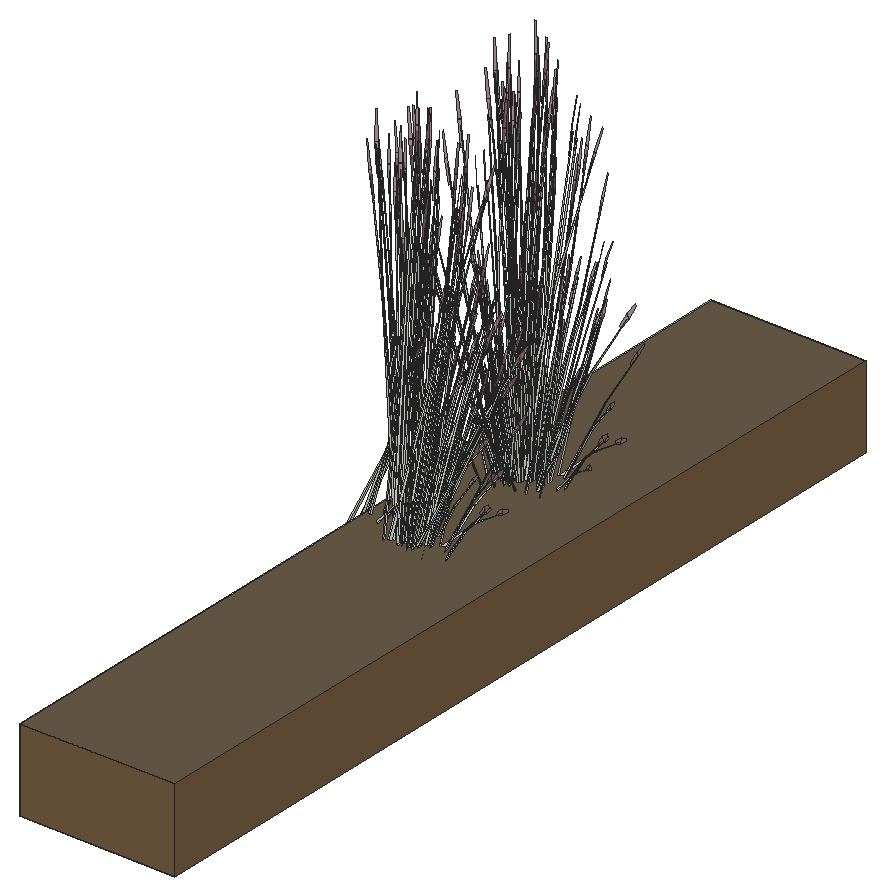
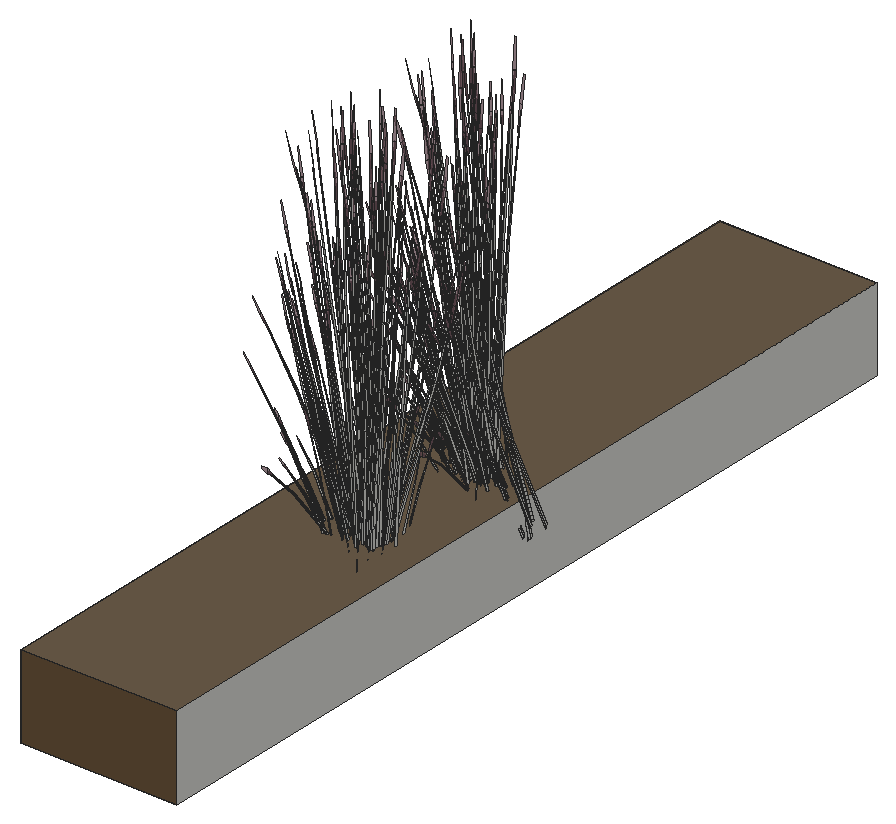
# SketchUp Ruby script. Lengths in inches.
U = 1.inch
M = Sketchup.active_model
def pt(a) = Geom::Point3d.new(a.map { |v| v * U })
def face(e, loops, mat)
  f = e.add_face(loops[0].map { |a| pt(a) })
  loops[1..].each { |l| e.add_face(l.map { |a| pt(a) }).erase! }
  f.material = f.back_material = mat if mat
  f
end
# faces: each face lists its corners as indices into pts; further lists are holes
def faces(e, pts, list, mat = nil) = list.each { |f| face(e, (f[0].is_a?(Array) ? f : [f]).map { |l| l.map { |i| pts[i] } }, mat) }
# xy, xz, yz: faces in a plane at the given z, y or x. An outline is a flat list of corners, or four numbers for a rectangle; further outlines are holes
def ring(l) = l.size == 4 ? [[l[0], l[1]], [l[2], l[1]], [l[2], l[3]], [l[0], l[3]]] : l.each_slice(2).to_a
def flat(e, list, mat, &to3) = list.each { |f| face(e, (f[0].is_a?(Array) ? f : [f]).map { |l| ring(l).map { |u, v| to3.(u, v) } }, mat) }
def xy(e, z, list, mat = nil) = flat(e, list, mat) { |x, y| [x, y, z] }
def xz(e, y, list, mat = nil) = flat(e, list, mat) { |x, z| [x, y, z] }
def yz(e, x, list, mat = nil) = flat(e, list, mat) { |y, z| [x, y, z] }
def lines(e, pts, list) = list.each { |a, b| e.add_line(pt(pts[a]), pt(pts[b])) }
# prism: a flat outline (further loops are holes) pulled along v
def prism(e, loops, v, mat = nil)
  f = face(e, loops, mat); d = Geom::Vector3d.new(v.map { |x| x * U })
  f.pushpull(f.normal.samedirection?(d) ? d.length : -d.length)
end
def box(e, o, s, mat = nil) = prism(e, [[o, [o[0] + s[0], o[1], o[2]], [o[0] + s[0], o[1] + s[1], o[2]], [o[0], o[1] + s[1], o[2]]]], [0, 0, s[2]], mat)
def at(x, y, z, deg = 0) = Geom::Transformation.translation(pt([x, y, z])) * Geom::Transformation.rotation(ORIGIN, Z_AXIS, deg.degrees)
def axes(o, x, y, z) = Geom::Transformation.new([*x, 0, *y, 0, *z, 0, *pt(o).to_a, 1])
def part(name) = M.definitions.add(name)
# library, detail: a bought-in or finely detailed component or shape, given as its bounding box
def library(name, o, s) = part(name).tap { |d| box(d.entities, o, s) }
def detail(e, o, s) = box(e.add_group.entities, o, s)
def put(e, d, t, mat = nil) = e.add_instance(d, t).tap { |i| i.material = mat if mat }
def group(e, t, mat = nil) = e.add_group.tap { |g| g.transformation = t; g.material = mat if mat }.entities
root = M.entities
M.materials.add("Forest_Floor_01_1K").color = [106, 91, 72]
M.materials.add("LightPink_Translucent").color = [144, 107, 117]
M.materials["LightPink_Translucent"].alpha = 0.75
M.materials.add("Soil_03_1K").color = [122, 96, 67]
c1 = part("blade")
p = [[2.15,0.21,22],[0,0.17,0],[0.09,0.45,0],[2.18,0.31,22],[2.29,0.31,22],[0.38,0.45,0],
  [2.48,0.24,33],[2.49,0.24,33],[2.48,0.22,33]]
faces(c1.entities,p,[[0,1,2,3],[4,5,2,3],[6,3,4,7],[8,0,3,6]])
c2 = part("seeds")
p = [[0.3,-0.1,1.38],[-0.01,-0.03,1.59],[-0.01,-0.03,0.03],[0.14,-0.07,-0.07],[0.29,-0.03,3],[0.15,0.01,3.11]]
faces(c2.entities,p,[[0,1,2,3],[1,0,4,5]],"LightPink_Translucent")
c3 = part("blade with seeds")
put(c3.entities,c1,at(0,0,0))
put(c3.entities,c2,axes([2.4,0.25,30.99],[1.5799,-0.05474,1.17369],[-0.12525,1.92788,0.29478],[-0.07173,-0.02425,1.56792]))
xy(root,-6,[[499.43,101.25,522.8,231.83]])
xy(root,6.51,[[499.43,101.25,522.8,231.83]],"Forest_Floor_01_1K")
xz(root,101.25,[[499.43,-6,522.8,6.51]],"Soil_03_1K")
xz(root,231.83,[[499.43,-6,522.8,6.51]],"Soil_03_1K")
yz(root,499.43,[[101.25,-6,231.83,6.51]])
yz(root,522.8,[[101.25,-6,231.83,6.51]],"Soil_03_1K")
put(root,c3,axes([506.22,163.54,1.55],[-0.62999,0.55453,0.45755],[-0.74845,-0.4895,0.17955],[0.15188,-0.05534,1.58856]))
put(root,c3,axes([506.91,164.54,1.49],[-0.70674,-0.52593,-0.06131],[0.70717,-0.52625,0],[-0.02468,-0.01837,1.75571]))
put(root,c3,axes([505.13,162.63,1.67],[-0.21949,0.60727,0.17642],[-0.8032,-0.17185,0.35086],[0.13875,-0.00296,1.60407]))
put(root,c3,axes([509.12,164.61,4.24],[-0.63144,-0.17046,0.35414],[0.18417,-0.49731,-0.4572],[0.25423,-0.0456,0.87481]))
put(root,c3,axes([504.8,163.12,0.79],[-0.74787,0.24464,1.28929],[-0.23804,-0.70192,0.50096],[0.45924,0.01168,1.46642]))
put(root,c3,axes([506.81,163.31,1.81],[0.14658,-0.54532,0.1448],[0.71613,0.09466,-0.41347],[0.13033,0.05599,1.26744]))
put(root,c3,axes([505.57,164.6,1.55],[0.96033,0.12874,0.45755],[-0.19544,0.7271,0.17955],[-0.14034,-0.07021,1.58856]))
put(root,c3,axes([510.64,164.07,0.6875],[-0.03971,-0.09277,1.76342],[0.27541,-0.54264,-0.26939],[0.27782,-0.00781,0.30037]))
put(root,c3,axes([506.5,163.45,1.91],[-0.45644,-0.51287,0.44739],[0.69137,-0.36116,-0.21531],[0.14771,0.06346,1.43643]))
put(root,c3,axes([505.05,165.76,1.67],[0.81646,-0.16218,0.17642],[0.20161,0.60355,0.35086],[-0.07282,-0.08794,1.60407]))
put(root,c3,axes([506.73,163.48,1.86],[0.76714,-0.40567,-0.29095],[0.51013,0.57321,-0.50002],[0.18927,0.05821,1.59708]))
put(root,c3,axes([509.78,164.55,3.72],[0.63144,0.17046,-0.35414],[-0.18417,0.49731,0.4572],[0.25423,-0.0456,0.87481]))
put(root,c3,axes([508.67,162.41,1.21],[0.7111,0.30552,-0.49651],[-0.42504,0.54784,0],[0.16196,0.06958,1.57504]))
put(root,c3,axes([507.32,164.15,1.4],[0.85008,0,0],[0,0.63259,0],[0,0,1.78407]))
put(root,c3,axes([500.02,166.56,3.91],[0.10543,-0.09307,1.74944],[-0.13495,-0.57092,-0.27667],[0.26455,-0.10825,0.14031]))
put(root,c3,axes([507.56,162.66,1.67],[-0.81646,0.16218,0.17642],[-0.20161,-0.60355,0.35086],[0.07282,0.08794,1.60407]))
put(root,c3,axes([508.0625,163.9375,3.07],[-0.31515,0.01384,1.71376],[0.20907,-0.5998,0.13857],[0.44912,0.0371,0.73262]))
put(root,c3,axes([508.47,162.63,1.22],[0.17848,0.53243,-0.30978],[-0.70886,0.15119,0.30978],[0.1429,0.0614,1.38974]))
put(root,c3,axes([509.69,164.76,3.92],[0.27906,0.41663,0.0643],[-0.50888,0.20393,0.50621],[0.22432,-0.04024,0.77189]))
put(root,c3,axes([507.04,163.83,1.57],[-0.96033,-0.12874,0.49198],[0.19544,-0.7271,0.19306],[0.14034,0.07021,1.70813]))
put(root,c3,axes([509.64,164.61,3.93],[-0.21466,0.55714,0.48003],[-0.70573,-0.19051,0.3958],[0.27753,-0.03348,0.9933]))
put(root,c3,axes([506.28,165.62,1.4],[-0.24791,-0.5268,0],[0.70791,-0.18448,0],[0,0,1.54371]))
put(root,c3,axes([507.21,165.55,1.38],[0.79769,-0.20732,-0.19198],[0.2803,0.59721,0.00008],[0.08805,-0.02292,1.73897]))
put(root,c3,axes([507.48,165.8,1.67],[0.21949,-0.60727,0.17642],[0.8032,0.17185,0.35086],[-0.13875,0.00296,1.60407]))
put(root,c3,axes([507.3,164.42,1.41],[0.53038,0.39469,0],[-0.53038,0.39469,0],[0,0,1.69266]))
put(root,c3,axes([508.74,164.25,1.67],[-0.59697,-0.44509,0.17642],[0.60159,-0.4317,0.35086],[-0.06593,0.0909,1.60407]))
put(root,c3,axes([507.63,163.58,1.25],[0.79037,0.10018,-0.62353],[-0.16679,0.61794,-0.16365],[0.23587,0.07488,1.37633]))
put(root,c3,axes([511.125,164.65,1.96],[-0.46945,0.10088,1.1486],[0.22097,-0.4169,0.84392],[0.24904,0.02853,0.25299]))
put(root,c3,axes([506.1,165.86,1.39],[-0.76598,-0.27433,0],[0.36864,-0.57001,0],[0,0,1.62707]))
put(root,c3,axes([498.67,167.11,1.17],[-0.48937,0.07333,1.41583],[-0.07789,-0.58369,0.08104],[0.34275,-0.08835,0.80566]))
put(root,c3,axes([507.29,163.96,1.91],[0.36864,-0.55059,0.44739],[0.76598,0.26498,-0.21531],[0,0.12692,1.43643]))
put(root,c3,axes([510.91,166.42,3.9],[-0.0687,-0.05349,1.77383],[0.15029,-0.57341,-0.16761],[0.27062,-0.03664,0.31391]))
put(root,c3,axes([507.15,164.27,1.48],[0,0.70667,-0.05637],[-0.95008,0,0],[0,0.02221,1.79368]))
put(root,c3,axes([497.78,167.15,4.17],[0.66765,-0.26986,-0.71045],[0.37208,0.55551,0.08574],[0.32259,-0.0631,1.00501]))
put(root,c3,axes([507.22,163.77,1.4],[0.45644,0.51287,-0.44739],[-0.69137,0.36116,0.21531],[0.14771,0.06346,1.43643]))
put(root,c3,axes([510.31,165.94,3.12],[-0.14542,-0.51365,-0.03492],[0.68734,-0.11809,-0.15832],[0.14353,0.03256,0.52218]))
put(root,c3,axes([508.53,165.92,4.23],[0.04068,-0.62141,-0.1216],[0.77029,0.01698,-0.67495],[0.29667,0.04317,1.02557]))
put(root,c3,axes([509.23,164.26,1.67],[0,-0.61104,0.49651],[0.85008,0,0],[0,0.13917,1.57504]))
put(root,c3,axes([507.1,164.72,1.91],[0.82508,-0.03772,0.44739],[0.07462,0.62614,-0.21531],[-0.14771,0.06346,1.43643]))
put(root,c3,axes([507.61,164.08,1.81],[0.70791,-0.1782,0.1448],[0.24791,0.50885,-0.41347],[0,0.11199,1.26744]))
put(root,c3,axes([508.41,165.68,4.24],[-0.43232,-0.38257,0.35414],[0.49364,-0.36215,-0.4572],[0.25081,0.0551,0.87481]))
put(root,c3,axes([510.24,165.32,1.78],[-0.18299,-0.15028,1.43002],[0.23809,-0.49714,-0.30754],[0.37023,0.06735,0.61141]))
put(root,c3,axes([499.2,166.72,0.6875],[-0.03971,-0.09277,1.76342],[0.27541,-0.54264,-0.26939],[0.27782,-0.00781,0.30037]))
put(root,c3,axes([506.97,165.87,1.4],[0.76598,0.27433,0],[-0.36864,0.57001,0],[0,0,1.74954]))
put(root,c3,axes([509.2,165.55,3.91],[0.16299,-0.01033,1.74944],[0.44707,-0.47471,-0.27667],[0.28992,0.06266,0.14031]))
put(root,c3,axes([507.11,164.99,1.81],[0.56134,0.36712,0.1448],[-0.46823,0.41419,-0.41347],[-0.13033,0.05599,1.26744]))
put(root,c3,axes([498.35,167.2,3.72],[0.63144,0.17046,-0.35414],[-0.18417,0.49731,0.4572],[0.25423,-0.0456,0.87481]))
put(root,c3,axes([508.5625,165.625,4.17],[0.75952,0.01471,-0.71045],[-0.05101,0.61953,0.08574],[0.32177,0.06538,1.00501]))
put(root,c3,axes([507.71,166.12,1.67],[0.7111,-0.30552,0.49651],[0.42504,0.54784,0],[-0.16196,0.06958,1.57504]))
put(root,c3,axes([506.7,165.64,1.48],[0.33034,0.70197,-0.06012],[-0.94388,0.24598,0],[0.01154,0.02451,1.72173]))
put(root,c3,axes([496.625,166.59,3.07],[-0.31515,0.01384,1.71376],[0.20907,-0.5998,0.13857],[0.44912,0.0371,0.73262]))
put(root,c3,axes([509.81,164.37,1.57],[0.95008,0,0],[0,0.68292,-0.51607],[0,0.15554,1.63711]))
put(root,c3,axes([509.43,164.72,1.39],[-0.94962,-0.00489,-0.04976],[0,-0.68292,0.49943],[-0.02984,0.15546,1.58352]))
put(root,c3,axes([507.37,164.125,1.86],[0.85568,0.29155,-0.29095],[-0.41201,0.61537,-0.50002],[0.02689,0.15109,1.59708]))
put(root,c3,axes([509.02,165.88,3.72],[0.43232,0.38257,-0.35414],[-0.49364,0.36215,0.4572],[0.25081,0.0551,0.87481]))
put(root,c3,axes([509.23,164.82,1.22],[-0.53038,0.38124,-0.30978],[-0.53038,-0.38124,0.30978],[0,0.1228,1.38974]))
put(root,c3,axes([506.94,164.86,1.86],[0.08854,0.69723,-0.29095],[-0.92215,0.04216,-0.50002],[-0.16238,0.09287,1.59708]))
put(root,c3,axes([508.8,166.03,3.92],[-0.03826,0.46465,0.0643],[-0.57772,-0.01274,0.50621],[0.2213,0.04862,0.77189]))
put(root,c3,axes([507.28,164.58,1.4],[-0.36864,0.55059,-0.44739],[-0.76598,-0.26498,0.21531],[0,0.12692,1.43643]))
put(root,c3,axes([508.85,165.88,3.93],[-0.56024,0.40262,0.48003],[-0.48318,-0.42758,0.3958],[0.26285,0.07427,0.9933]))
put(root,c3,axes([499.6875,167.3,1.96],[-0.46945,0.10088,1.1486],[0.22097,-0.4169,0.84392],[0.24904,0.02853,0.25299]))
put(root,c3,axes([507.07,166.35,4.24],[-0.11735,-0.49217,0.35414],[0.67083,-0.12996,-0.4572],[0.18018,0.14104,0.87481]))
put(root,c3,axes([507.3,166.16,1.52],[0.95122,0.19861,0.30756],[-0.23797,0.7099,-0.36492],[-0.15744,0.08885,1.64885]))
put(root,c3,axes([499.47,169.07,3.9],[-0.0687,-0.05349,1.77383],[0.15029,-0.57341,-0.16761],[0.27062,-0.03664,0.31391]))
put(root,c3,axes([509.59,164.83,1.21],[0,0.61104,-0.49651],[-0.85008,0,0],[0,0.13917,1.57504]))
put(root,c3,axes([507.47,164.9,3.07],[-0.28223,-0.10528,1.71376],[0.58406,-0.44165,0.13857],[0.36402,0.19924,0.73262]))
put(root,c3,axes([507.52,163.51,3.67],[-0.65655,-0.31748,1.38283],[0.69326,-0.49431,0.59665],[0.21183,0.29789,1.33663]))
put(root,c3,axes([508.51,166.1,1.96],[-0.4278,-0.1757,1.1486],[0.5524,-0.17852,0.84392],[0.14899,0.15122,0.25299]))
put(root,c3,axes([507.01,166.6,4.23],[0.45276,-0.52302,-0.1216],[0.65568,0.30132,-0.67495],[0.22792,0.14777,1.02557]))
put(root,c3,axes([498.81,167.97,1.78],[-0.18299,-0.15028,1.43002],[0.23809,-0.49714,-0.30754],[0.37023,0.06735,0.61141]))
put(root,c3,axes([504.03,165.89,4.24],[0.5141,-0.32171,0.35414],[0.48666,0.36734,-0.4572],[-0.07405,0.18664,0.87481]))
put(root,c3,axes([507.875,166.55,1.57],[0.47504,0.61229,0],[-0.79476,0.34146,-0.51607],[-0.18101,0.07777,1.63711]))
put(root,c3,axes([506.42,167.03,3.9],[0.00225,-0.07398,1.77383],[0.65113,-0.32638,-0.16761],[0.22617,0.1165,0.31391]))
put(root,c3,axes([508.63,166.75,0.6875],[0.05536,-0.08822,1.76342],[0.69692,-0.25981,-0.26939],[0.21129,0.13447,0.30037]))
put(root,c3,axes([507.47,164.12,2.03],[-0.02076,-0.57531,1.41272],[0.93937,0.14913,0.59816],[-0.22217,0.31481,1.3335]))
put(root,c3,axes([507.71,164.75,1.29],[0.2786,0.55945,-0.69212],[-0.80253,0.20149,-0.18165],[0.03079,0.18945,1.52773]))
put(root,c3,axes([507.55,166.34,3.875],[0.74975,-0.14525,-0.51099],[0.13115,0.55007,-0.3958],[0.20138,0.15763,0.97773]))
put(root,c3,axes([505.47,166.42,4.24],[0.22906,-0.4699,0.35414],[0.66828,0.13705,-0.4572],[0.06128,0.18919,0.87481]))
put(root,c3,axes([508.58,166.9,1.86],[-0.48723,-0.01916,1.0506],[0.32177,-0.40701,0.58006],[0.19248,0.1446,0.8241]))
put(root,c3,axes([507.18,166.79,3.92],[-0.34533,0.38816,0.0643],[-0.49176,-0.22599,0.50621],[0.15898,0.12445,0.77189]))
put(root,c3,axes([497.125,168.27,4.17],[0.75952,0.01471,-0.71045],[-0.05101,0.61953,0.08574],[0.32177,0.06538,1.00501]))
put(root,c3,axes([506.37,168.1,4.84],[0.52505,-0.35054,-0.06488],[0.48109,0.38392,-0.29416],[0.03387,0.10878,0.97024]))
put(root,c3,axes([507.32,166.68,3.93],[-0.75571,0.14023,0.48003],[-0.13115,-0.55007,0.3958],[0.17773,0.16212,0.9933]))
put(root,c3,axes([506.99,165.91,1.78],[0.01341,-0.20255,1.43002],[0.64074,-0.22625,-0.30754],[0.1978,0.24243,0.61141]))
put(root,c3,axes([505.26,166.85,3.92],[-0.55987,0.20767,0.0643],[-0.27403,-0.37869,0.50621],[0.05407,0.16693,0.77189]))
put(root,c3,axes([503.7,165.98,4.59],[0.83505,0.03027,-0.13498],[-0.02282,0.57322,-0.74919],[-0.05801,0.22077,1.13838]))
put(root,c3,axes([505.24,166.62,4.23],[0.74352,-0.28449,-0.1216],[0.36538,0.50492,-0.67495],[0.0981,0.21277,1.02557]))
put(root,c3,axes([505.46,166.81,4.26],[-0.74868,-0.15974,0.53283],[0.25601,-0.52518,0.43934],[0.04499,0.20653,1.10256]))
put(root,c3,axes([505.38,166.73,0.6875],[0.12297,-0.03325,1.76342],[0.73967,0.18301,-0.26939],[0.02163,0.20626,0.30037]))
put(root,c3,axes([503.68,166.82,2.02],[0.69024,-0.1082,0.06507],[0.15868,0.43593,-0.86304],[-0.04376,0.22067,0.7736]))
put(root,c3,axes([505.88,166.6,3.875],[0.7469,0.15318,-0.51099],[-0.25601,0.52518,-0.3958],[0.06849,0.21144,0.97773]))
put(root,c3,axes([506.31,165.51,3.07],[-0.17368,-0.19618,1.71376],[0.80256,-0.16516,0.13857],[0.18139,0.30799,0.73262]))
put(root,c3,axes([505.54,166.92,3.72],[-0.22906,0.4699,-0.35414],[-0.66828,-0.13705,0.4572],[0.06128,0.18919,0.87481]))
put(root,c3,axes([504.89,165.61,3.07],[-0.0186,-0.23452,1.71376],[0.80601,0.15558,0.13857],[-0.04985,0.33422,0.73262]))
put(root,c3,axes([505.61,166.5,4.17],[0.36264,0.49684,-0.71045],[-0.74649,0.27689,0.08574],[0.0848,0.24006,1.00501]))
put(root,c3,axes([505.07,167.75,3.91],[0.09631,0.0984,1.74944],[0.77725,0.03866,-0.27667],[0.07816,0.217,0.14031]))
put(root,c3,axes([507.76,183.48,1.78],[-0.21597,0.12368,1.43002],[-0.64681,-0.21647,-0.30754],[0.1199,-0.26922,0.61141]))
put(root,c3,axes([506.77,183.92,4.17],[-0.36264,-0.49684,-0.71045],[0.74649,-0.27689,0.08574],[-0.0848,-0.24006,1.00501]))
put(root,c3,axes([506.15,182.8125,0.6875],[-0.12744,0.02202,1.76342],[-0.70477,-0.24781,-0.26939],[0.01183,-0.2067,0.30037]))
put(root,c3,axes([508.28,184.4,4.17],[0.01977,-0.56521,-0.71045],[0.83252,0.03796,0.08574],[0.08786,-0.23945,1.00501]))
put(root,c3,axes([509.44,183.52,3.91],[-0.00733,-0.12161,1.74944],[-0.61946,-0.35147,-0.27667],[0.09577,-0.21306,0.14031]))
put(root,c3,axes([506.84,183.49,3.72],[0.22906,-0.4699,-0.35414],[0.66828,0.13705,0.4572],[-0.06128,-0.18919,0.87481]))
put(root,c3,axes([507.34,184.11,3.07],[-0.14147,0.21002,1.71376],[-0.59349,-0.43464,0.13857],[0.26773,-0.27089,0.73262]))
put(root,c3,axes([509.28,183.08,3.9],[-0.07716,0.04667,1.77383],[-0.75601,-0.15746,-0.16761],[-0.02737,-0.20368,0.31391]))
put(root,c3,axes([506.5,183.82,3.875],[-0.7469,-0.15318,-0.51099],[0.25601,-0.52518,-0.3958],[-0.06849,-0.21144,0.97773]))
put(root,c3,axes([506.96,182.5,1.96],[0.09747,0.35631,1.1486],[-0.54071,-0.19735,0.84392],[0.05818,-0.18244,0.25299]))
put(root,c3,axes([508.11,184.21,3.875],[-0.54391,-0.41056,-0.51099],[0.57458,-0.35956,-0.3958],[0.08276,-0.2086,0.97773]))
put(root,c3,axes([506.92,183.6,3.93],[0.74868,0.15974,0.48003],[-0.25601,0.52518,0.3958],[-0.04499,-0.20653,0.9933]))
put(root,c3,axes([507.14,183.79,4.23],[-0.74352,0.28449,-0.1216],[-0.36538,-0.50492,-0.67495],[-0.0981,-0.21277,1.02557]))
put(root,c3,axes([508.68,184.43,4.23],[-0.83505,-0.03027,-0.1216],[0.02282,-0.57322,-0.67495],[0.05801,-0.22077,1.02557]))
put(root,c3,axes([508.625,184.0625,3.72],[0.5141,-0.32171,-0.35414],[0.48666,0.36734,0.4572],[0.07405,-0.18664,0.87481]))
put(root,c3,axes([507.12,183.5625,3.92],[0.55987,-0.20767,0.0643],[0.27403,0.37869,0.50621],[-0.05407,-0.16693,0.77189]))
put(root,c3,axes([505.09,185.78,1.29],[-0.31203,-0.62659,-0.69835],[0.89884,-0.22566,-0.18329],[-0.03449,-0.21218,1.54149]))
put(root,c3,axes([509.27,183.87,0.6875],[-0.11372,-0.04814,1.76342],[-0.29211,-0.53779,-0.26939],[0.19706,-0.14594,0.30037]))
put(root,c3,axes([506.91,183.99,4.24],[-0.22906,0.4699,0.35414],[-0.66828,-0.13705,-0.4572],[-0.06128,-0.18919,0.87481]))
put(root,c3,axes([508.62,184.1875,3.93],[0.54105,0.41691,0.48003],[-0.57458,0.35956,0.3958],[0.0998,-0.1956,0.9933]))
put(root,c3,axes([508.82,184.23,3.92],[0.62439,0.02847,0.0643],[-0.01712,0.42991,0.50621],[0.06534,-0.16468,0.77189]))
put(root,c3,axes([508.36,184.52,4.24],[-0.5141,0.32171,0.35414],[-0.48666,-0.36734,-0.4572],[0.07405,-0.18664,0.87481]))
put(root,c3,axes([509.26,185.38,4.17],[0.39688,-0.48213,-0.71045],[0.69548,0.34264,0.08574],[0.23697,-0.17468,1.00501]))
put(root,c3,axes([504.97,183.98,1.57],[-0.47504,-0.61229,0],[0.79476,-0.34146,-0.51607],[0.18101,-0.07777,1.63711]))
put(root,c3,axes([509.24,185.16,3.875],[-0.19519,-0.55794,-0.51099],[0.73919,-0.0976,-0.3958],[0.21183,-0.14986,0.97773]))
put(root,c3,axes([506.01,183.24,1.32],[-0.52505,0.35054,-0.03893],[-0.48109,-0.38392,-0.17649],[-0.03387,-0.10878,0.58215]))
put(root,c3,axes([509.59,185.56,4.23],[-0.70283,-0.33692,-0.1216],[0.40491,-0.48793,-0.67495],[0.19857,-0.16961,1.02557]))
put(root,c3,axes([505.62,183.88,1.21],[0.7111,-0.30552,-0.49651],[0.42504,0.54784,0],[0.16196,-0.06958,1.57504]))
put(root,c3,axes([509.84,184.94,1.78],[-0.27143,-0.0181,1.43002],[-0.27808,-0.48551,-0.30754],[0.33346,-0.13735,0.61141]))
put(root,c3,axes([511.32,185.41,3.9],[-0.09924,-0.00464,1.77383],[-0.4121,-0.49725,-0.16761],[0.1655,-0.1635,0.31391]))
put(root,c3,axes([506.46,185.14,1.25],[0.51177,-0.45928,-0.62353],[0.63575,0.41646,-0.16365],[0.20507,-0.11457,1.37633]))
put(root,c3,axes([510.15,184.05,1.96],[-0.25308,0.31105,1.1486],[-0.21753,-0.4179,0.84392],[0.20902,-0.10472,0.25299]))
put(root,c3,axes([509.79,185.22,3.72],[0.66138,-0.08733,-0.35414],[0.17464,0.49921,0.4572],[0.18953,-0.13408,0.87481]))
put(root,c3,axes([505.57,185.94,1.4],[0.36864,-0.55059,-0.44739],[0.76598,0.26498,0.21531],[0,-0.12692,1.43643]))
put(root,c3,axes([505.9,185.67,1.86],[-0.08854,-0.69723,-0.29095],[0.92215,-0.04216,-0.50002],[0.16238,-0.09287,1.59708]))
put(root,c3,axes([503.62,185.71,1.22],[0.53038,-0.38124,-0.30978],[0.53038,0.38124,0.30978],[0,-0.1228,1.38974]))
put(root,c3,axes([509.25,185.51,4.24],[-0.66138,0.08733,0.35414],[-0.17464,-0.49921,-0.4572],[0.18953,-0.13408,0.87481]))
put(root,c3,axes([505.48,186.4,1.86],[-0.85568,-0.29155,-0.29095],[0.41201,-0.61537,-0.50002],[-0.02689,-0.15109,1.59708]))
put(root,c3,axes([505.78,184.125,1.22],[0.70886,0.15119,-0.30978],[-0.17848,0.53243,0.30978],[0.1429,-0.0614,1.38974]))
put(root,c3,axes([509.85,185.43,3.92],[0.52161,0.25698,0.0643],[-0.30368,0.36595,0.50621],[0.16723,-0.11831,0.77189]))
put(root,c3,axes([509.7,185.32,3.93],[0.18844,0.56237,0.48003],[-0.73919,0.0976,0.3958],[0.21785,-0.13226,0.9933]))
put(root,c3,axes([511.7,186.01,3.91],[0.10543,-0.09307,1.74944],[-0.13495,-0.57092,-0.27667],[0.26455,-0.10825,0.14031]))
put(root,c3,axes([506.03,186.22,1.625],[0.8561,0.29616,0.24065],[-0.41201,0.61537,0.50002],[0,-0.14185,1.60543]))
put(root,c3,axes([505.75,185.8,1.91],[-0.82508,0.03772,0.44739],[-0.07462,-0.62614,-0.21531],[0.14771,-0.06346,1.43643]))
put(root,c3,axes([509.62,186.87,4.23],[-0.38229,-0.5533,-0.1216],[0.6785,-0.2719,-0.67495],[0.28593,-0.073,1.02557]))
put(root,c3,axes([509.59,186.4,3.875],[0.20584,-0.55581,-0.51099],[0.70573,0.19051,-0.3958],[0.28414,-0.05097,0.97773]))
put(root,c3,axes([508.47,184.13,1.57],[0.47504,-0.61229,0],[0.79476,0.34146,-0.51607],[0.18101,0.07777,1.63711]))
put(root,c3,axes([505.72,186.03,1.55],[0.33034,0.68327,0.45755],[-0.94388,0.2376,0.17955],[0.01154,-0.12555,1.58856]))
put(root,c3,axes([510.34,186.55,1.17],[-0.48937,0.07333,1.41583],[-0.07789,-0.58369,0.08104],[0.34275,-0.08835,0.80566]))
put(root,c3,axes([511.23,186.04,1.45],[-0.47106,-0.39072,-0.06488],[0.51591,-0.35801,-0.29416],[0.14618,-0.02521,0.97024]))
put(root,c3,axes([505.55,186.57,1.91],[-0.36864,0.55059,0.44739],[-0.76598,-0.26498,-0.21531],[0,-0.12692,1.43643]))
put(root,c3,axes([506.91,186.09,1.4],[0,-0.70701,0],[0.95008,0,0],[0,0,1.79456]))
put(root,c3,axes([508.06,184.45,1.67],[-0.7111,-0.30552,0.49651],[0.42504,-0.54784,0],[0.16196,0.06958,1.57504]))
put(root,c3,axes([509.45,186.6,4.17],[0.66765,-0.26986,-0.71045],[0.37208,0.55551,0.08574],[0.32259,-0.0631,1.00501]))
put(root,c3,axes([506.46,185.64,1.55],[-0.62999,0.55453,0.45755],[-0.74845,-0.4895,0.17955],[0.15188,-0.05534,1.58856]))
put(root,c3,axes([507.15,186.64,1.49],[-0.70674,-0.52593,-0.06131],[0.70717,-0.52625,0],[-0.02468,-0.01837,1.75571]))
put(root,c3,axes([505.36,184.73,1.67],[-0.21949,0.60727,0.17642],[-0.8032,-0.17185,0.35086],[0.13875,-0.00296,1.60407]))
put(root,c3,axes([509.35,186.71,4.24],[-0.63144,-0.17046,0.35414],[0.18417,-0.49731,-0.4572],[0.25423,-0.0456,0.87481]))
put(root,c3,axes([505.03,185.22,0.79],[-0.74787,0.24464,1.28929],[-0.23804,-0.70192,0.50096],[0.45924,0.01168,1.46642]))
put(root,c3,axes([507.04,185.4,1.81],[0.14658,-0.54532,0.1448],[0.71613,0.09466,-0.41347],[0.13033,0.05599,1.26744]))
put(root,c3,axes([505.8,186.7,1.55],[0.96033,0.12874,0.45755],[-0.19544,0.7271,0.17955],[-0.14034,-0.07021,1.58856]))
put(root,c3,axes([510.875,186.17,0.6875],[-0.03971,-0.09277,1.76342],[0.27541,-0.54264,-0.26939],[0.27782,-0.00781,0.30037]))
put(root,c3,axes([506.74,185.55,1.91],[-0.45644,-0.51287,0.44739],[0.69137,-0.36116,-0.21531],[0.14771,0.06346,1.43643]))
put(root,c3,axes([505.29,187.86,1.67],[0.81646,-0.16218,0.17642],[0.20161,0.60355,0.35086],[-0.07282,-0.08794,1.60407]))
put(root,c3,axes([506.97,185.58,1.86],[0.76714,-0.40567,-0.29095],[0.51013,0.57321,-0.50002],[0.18927,0.05821,1.59708]))
put(root,c3,axes([510.02,186.65,3.72],[0.63144,0.17046,-0.35414],[-0.18417,0.49731,0.4572],[0.25423,-0.0456,0.87481]))
put(root,c3,axes([508.9,184.5,1.21],[0.7111,0.30552,-0.49651],[-0.42504,0.54784,0],[0.16196,0.06958,1.57504]))
put(root,c3,axes([507.55,186.25,1.4],[0.85008,0,0],[0,0.63259,0],[0,0,1.78407]))
put(root,c3,axes([507.79,184.76,1.67],[-0.81646,0.16218,0.17642],[-0.20161,-0.60355,0.35086],[0.07282,0.08794,1.60407]))
put(root,c3,axes([508.3,186.04,3.07],[-0.31515,0.01384,1.71376],[0.20907,-0.5998,0.13857],[0.44912,0.0371,0.73262]))
put(root,c3,axes([508.7,184.73,1.22],[0.17848,0.53243,-0.30978],[-0.70886,0.15119,0.30978],[0.1429,0.0614,1.38974]))
put(root,c3,axes([509.93,186.86,3.92],[0.27906,0.41663,0.0643],[-0.50888,0.20393,0.50621],[0.22432,-0.04024,0.77189]))
put(root,c3,axes([507.28,185.92,1.57],[-0.96033,-0.12874,0.49198],[0.19544,-0.7271,0.19306],[0.14034,0.07021,1.70813]))
put(root,c3,axes([509.87,186.71,3.93],[-0.21466,0.55714,0.48003],[-0.70573,-0.19051,0.3958],[0.27753,-0.03348,0.9933]))
put(root,c3,axes([506.51,187.72,1.4],[-0.24791,-0.5268,0],[0.70791,-0.18448,0],[0,0,1.54371]))
put(root,c3,axes([507.44,187.64,1.38],[0.79769,-0.20732,-0.19198],[0.2803,0.59721,0.00008],[0.08805,-0.02292,1.73897]))
put(root,c3,axes([507.72,187.89,1.67],[0.21949,-0.60727,0.17642],[0.8032,0.17185,0.35086],[-0.13875,0.00296,1.60407]))
put(root,c3,axes([507.53,186.52,1.41],[0.53038,0.39469,0],[-0.53038,0.39469,0],[0,0,1.69266]))
put(root,c3,axes([508.97,186.34,1.67],[-0.59697,-0.44509,0.17642],[0.60159,-0.4317,0.35086],[-0.06593,0.0909,1.60407]))
put(root,c3,axes([507.87,185.67,1.25],[0.79037,0.10018,-0.62353],[-0.16679,0.61794,-0.16365],[0.23587,0.07488,1.37633]))
put(root,c3,axes([511.36,186.75,1.96],[-0.46945,0.10088,1.1486],[0.22097,-0.4169,0.84392],[0.24904,0.02853,0.25299]))
put(root,c3,axes([506.34,187.96,1.39],[-0.76598,-0.27433,0],[0.36864,-0.57001,0],[0,0,1.62707]))
put(root,c3,axes([507.53,186.06,1.91],[0.36864,-0.55059,0.44739],[0.76598,0.26498,-0.21531],[0,0.12692,1.43643]))
put(root,c3,axes([511.14,188.52,3.9],[-0.0687,-0.05349,1.77383],[0.15029,-0.57341,-0.16761],[0.27062,-0.03664,0.31391]))
put(root,c3,axes([507.39,186.37,1.48],[0,0.70667,-0.05637],[-0.95008,0,0],[0,0.02221,1.79368]))
put(root,c3,axes([507.46,185.87,1.4],[0.45644,0.51287,-0.44739],[-0.69137,0.36116,0.21531],[0.14771,0.06346,1.43643]))
put(root,c3,axes([510.54,188.04,3.12],[-0.14542,-0.51365,-0.03492],[0.68734,-0.11809,-0.15832],[0.14353,0.03256,0.52218]))
put(root,c3,axes([508.76,188.02,4.23],[0.04068,-0.62141,-0.1216],[0.77029,0.01698,-0.67495],[0.29667,0.04317,1.02557]))
put(root,c3,axes([509.46,186.36,1.67],[0,-0.61104,0.49651],[0.85008,0,0],[0,0.13917,1.57504]))
put(root,c3,axes([507.33,186.82,1.91],[0.82508,-0.03772,0.44739],[0.07462,0.62614,-0.21531],[-0.14771,0.06346,1.43643]))
put(root,c3,axes([507.85,186.18,1.81],[0.70791,-0.1782,0.1448],[0.24791,0.50885,-0.41347],[0,0.11199,1.26744]))
put(root,c3,axes([508.64,187.78,4.24],[-0.43232,-0.38257,0.35414],[0.49364,-0.36215,-0.4572],[0.25081,0.0551,0.87481]))
put(root,c3,axes([510.48,187.42,1.78],[-0.18299,-0.15028,1.43002],[0.23809,-0.49714,-0.30754],[0.37023,0.06735,0.61141]))
put(root,c3,axes([507.21,187.97,1.4],[0.76598,0.27433,0],[-0.36864,0.57001,0],[0,0,1.74954]))
put(root,c3,axes([509.43,187.65,3.91],[0.16299,-0.01033,1.74944],[0.44707,-0.47471,-0.27667],[0.28992,0.06266,0.14031]))
